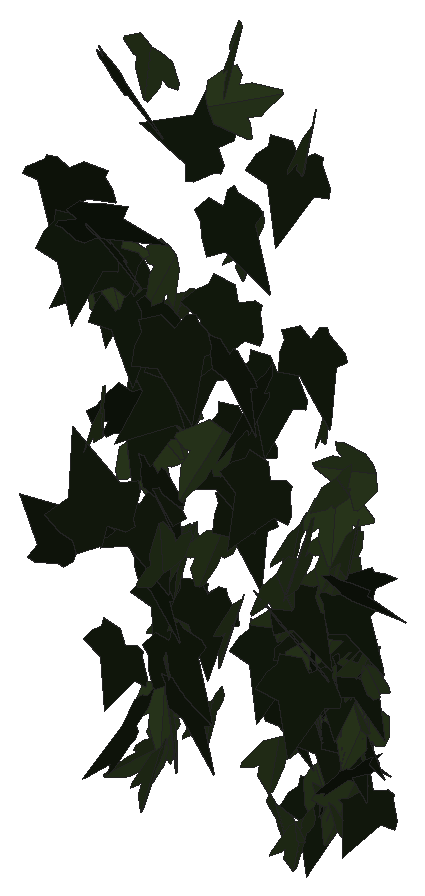
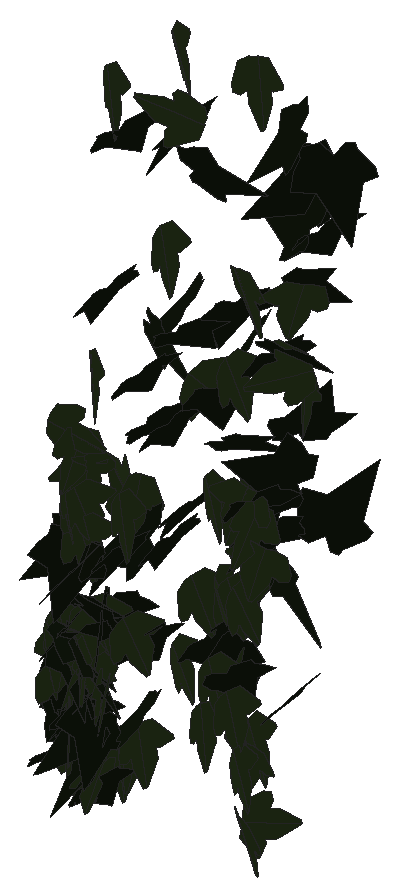
# SketchUp Ruby script. Lengths in inches.
U = 1.inch
M = Sketchup.active_model
def pt(a) = Geom::Point3d.new(a.map { |v| v * U })
def face(e, loops, mat)
  f = e.add_face(loops[0].map { |a| pt(a) })
  loops[1..].each { |l| e.add_face(l.map { |a| pt(a) }).erase! }
  f.material = f.back_material = mat if mat
  f
end
# faces: each face lists its corners as indices into pts; further lists are holes
def faces(e, pts, list, mat = nil) = list.each { |f| face(e, (f[0].is_a?(Array) ? f : [f]).map { |l| l.map { |i| pts[i] } }, mat) }
# xy, xz, yz: faces in a plane at the given z, y or x. An outline is a flat list of corners, or four numbers for a rectangle; further outlines are holes
def ring(l) = l.size == 4 ? [[l[0], l[1]], [l[2], l[1]], [l[2], l[3]], [l[0], l[3]]] : l.each_slice(2).to_a
def flat(e, list, mat, &to3) = list.each { |f| face(e, (f[0].is_a?(Array) ? f : [f]).map { |l| ring(l).map { |u, v| to3.(u, v) } }, mat) }
def xy(e, z, list, mat = nil) = flat(e, list, mat) { |x, y| [x, y, z] }
def xz(e, y, list, mat = nil) = flat(e, list, mat) { |x, z| [x, y, z] }
def yz(e, x, list, mat = nil) = flat(e, list, mat) { |y, z| [x, y, z] }
def lines(e, pts, list) = list.each { |a, b| e.add_line(pt(pts[a]), pt(pts[b])) }
# prism: a flat outline (further loops are holes) pulled along v
def prism(e, loops, v, mat = nil)
  f = face(e, loops, mat); d = Geom::Vector3d.new(v.map { |x| x * U })
  f.pushpull(f.normal.samedirection?(d) ? d.length : -d.length)
end
def box(e, o, s, mat = nil) = prism(e, [[o, [o[0] + s[0], o[1], o[2]], [o[0] + s[0], o[1] + s[1], o[2]], [o[0], o[1] + s[1], o[2]]]], [0, 0, s[2]], mat)
def at(x, y, z, deg = 0) = Geom::Transformation.translation(pt([x, y, z])) * Geom::Transformation.rotation(ORIGIN, Z_AXIS, deg.degrees)
def axes(o, x, y, z) = Geom::Transformation.new([*x, 0, *y, 0, *z, 0, *pt(o).to_a, 1])
def part(name) = M.definitions.add(name)
# library, detail: a bought-in or finely detailed component or shape, given as its bounding box
def library(name, o, s) = part(name).tap { |d| box(d.entities, o, s) }
def detail(e, o, s) = box(e.add_group.entities, o, s)
def put(e, d, t, mat = nil) = e.add_instance(d, t).tap { |i| i.material = mat if mat }
def group(e, t, mat = nil) = e.add_group.tap { |g| g.transformation = t; g.material = mat if mat }.entities
root = M.entities
M.materials.add("efeu1").color = [18, 25, 13]
M.materials.add("efeu2").color = [43, 57, 29]
c1 = part("ivyleaf_9")
p = [[1.54,2.16,1.25],[1.36,2.04,1.19],[-0.21,0.99,0.68],[-0.71,1.11,0.82],[-0.85,0.86,0.67],[-0.8,0.17,0.21],
  [-0.9,-0.01,0.1],[-0.67,-0.16,-0.02],[-0.08,-0.08,-0.05],[-0.03,-0.6,-0.4],[0.65,-0.88,-0.66],[0.83,-0.6,-0.49],
  [1.29,-0.42,-0.43],[1.8125,-0.07,-0.26],[1.21,0.44,0.15]]
faces(c1.entities,p,[[0,1,2,3,4,5,6,7,8,9,10,11,12,13,14]],"efeu1")
c2 = part("ivyleaf_10")
p = [[0,0.5,-0.03],[-0.0625,2.02,-0.43],[-0.19,2.01,-0.46],[-0.54,1.05,-0.29],[-0.52,0.625,-0.18],[-0.83,0.76,-0.28],
  [-1.16,0.64,-0.33],[-1.15,0.33,-0.24],[-0.77,-0.39,0.02],[-0.3,-0.51,0.16],[0.04,-0.48,0.23],[-0.02,2.01,-0.4375],
  [-0.06,2.01,-0.43],[0.04,-0.49,0.23],[0.67,-0.49,0.14],[1.38,0.36,-0.2],[1.375,0.51,-0.24],[0.81,0.65,-0.19],
  [0.62,0.59,-0.15],[0.6,1.09,-0.28],[0.5,1.23,-0.31]]
faces(c2.entities,p,[[0,1,2,3,4,5,6,7,8,9,10],[11,12,0,13,14,15,16,17,18,19,20]],"efeu2")
put(root,c1,axes([520.66,128.22,263.75],[-0.69365,-0.67132,-0.50091],[0.59941,0.05642,-0.90568],[0.58505,-0.85375,0.33402]))
put(root,c2,axes([520.98,130.83,246.47],[0.29708,-0.97872,0.03394],[0.01857,-0.02983,-1.02277],[0.97913,0.29752,0.0091]))
put(root,c2,axes([521.33,129.46,243.19],[-0.16336,0.40857,-0.92125],[-0.63007,-0.76979,-0.22967],[-0.78654,0.5318,0.37532]))
put(root,c2,axes([520.625,129.71,255.22],[0.91836,0.41459,0.34556],[0.25749,0.26283,-0.99965],[-0.47434,0.94536,0.12638]))
put(root,c2,axes([521,130.48,243.49],[0.86834,-0.61453,-0.01149],[-0.00928,0.00678,-1.0638],[0.61457,0.86839,0.00017]))
put(root,c2,axes([520.42,127.77,262.62],[0.32861,0.02903,1.02903],[0.67094,0.81321,-0.2372],[-0.78076,0.71104,0.22926]))
put(root,c1,axes([521.42,124.74,253.9],[0.43717,0.15121,1.08821],[-1.00297,-0.42313,0.46172],[0.44845,-1.09374,-0.02818]))
put(root,c2,axes([521.11,129.59,256.77],[-0.27803,-0.8168,-0.63572],[0.2236,0.59531,-0.86267],[1.01059,-0.35643,0.01598]))
put(root,c1,axes([520.92,128.12,247.9],[-0.16291,-0.90011,0.48411],[0.07985,-0.49993,-0.90266],[1.01891,-0.10474,0.14814]))
put(root,c1,axes([520.78,127.61,257.58],[0.30082,-0.03966,1.04482],[0.88917,0.58171,-0.23392],[-0.5501,0.91857,0.19325]))
put(root,c1,axes([521.27,129.5625,257.41],[-0.45716,-0.971,-0.0412],[0.00221,0.04449,-1.0731],[0.97187,-0.45685,-0.01694]))
put(root,c2,axes([521.58,129.97,253.13],[0.01932,-0.99801,0.34488],[0.00807,-0.34479,-0.9982],[1.05589,0.0209,0.00132]))
put(root,c1,axes([521.83,123.84,269.89],[0.53807,0.6933,-0.78828],[-0.48033,-0.62504,-0.8776],[-0.93345,0.72127,-0.0028]))
put(root,c2,axes([521.625,130.52,248.66],[-0.09822,-1.03062,0.0625],[0.00455,-0.06321,-1.03524],[1.03251,-0.09776,0.01051]))
put(root,c1,axes([521.91,126.54,265.4375],[-0.75241,-0.6843,0.4398],[-0.33722,-0.28278,-1.01692],[0.74025,-0.82436,-0.01624]))
put(root,c2,axes([521.37,126.44,265.23],[0.69116,0.81659,0.26113],[0.16323,0.20395,-1.0698],[-0.84164,0.71014,0.00697]))
put(root,c1,axes([521.13,126.97,272.73],[1.04056,-0.52413,-0.14017],[-0.12231,0.06878,-1.16509],[0.52859,1.04771,0.00636]))
put(root,c2,axes([521.61,129.64,257.48],[0.99003,0.20389,0.3712],[0.28016,0.3925,-0.9628],[-0.31761,0.98179,0.30782]))
put(root,c1,axes([521.94,130.27,249.84],[-0.53362,-0.89248,-0.01376],[0.01586,0.00655,-1.03979],[0.89245,-0.53376,0.01024]))
put(root,c1,axes([521.81,127.56,262.87],[-0.14103,-1.05826,-0.18674],[-0.01066,0.18971,-1.06704],[1.07456,-0.13701,-0.0351]))
put(root,c2,axes([521.95,129,245.91],[1.00038,-0.09883,0.26611],[0.26139,-0.05949,-1.00473],[0.11072,1.03346,-0.03239]))
put(root,c1,axes([521.99,124.53,266.91],[-0.20059,-1.13323,0.06662],[0.01428,-0.07017,-1.15055],[1.1351,-0.19938,0.02625]))
put(root,c2,axes([522.7,129.0625,252.7],[-0.23547,-0.99051,0.24855],[0.02076,-0.25966,-1.01512],[1.02101,-0.22315,0.07796]))
put(root,c2,axes([522.77,124.36,259.98],[0.27143,-0.85202,-0.61381],[-0.12326,0.60376,-0.89256],[1.04284,0.29312,0.05427]))
put(root,c1,axes([522.05,128.76,255.12],[0.49208,-0.89724,0.28373],[0.11153,-0.26232,-1.02295],[0.9344,0.50382,-0.02732]))
put(root,c2,axes([522.74,129.02,262.42],[0.02047,-1.05918,0.27122],[0.01003,-0.27107,-1.05937],[1.09331,0.02232,0.00464]))
put(root,c2,axes([522.9,130,249.48],[-0.01941,-1.03805,0.06821],[-0.01225,-0.06799,-1.03817],[1.04021,-0.02017,-0.01095]))
put(root,c1,axes([523.125,128.75,259.08],[-0.90533,-0.4986,0.31147],[-0.12446,-0.3964,-0.9963],[0.57456,-0.87149,0.27497]))
put(root,c1,axes([522.55,127.07,254.74],[-0.09928,-0.9378,-0.60059],[0.18853,0.58011,-0.93699],[1.09756,-0.18448,0.10663]))
put(root,c2,axes([522.92,128.41,245.82],[-0.53142,0.79284,-0.44341],[0.16062,-0.42361,-0.94994],[-0.8941,-0.54734,0.09289]))
put(root,c1,axes([522.3,124.9,267.1],[0.56545,-0.74923,0.57769],[0.45767,-0.3724,-0.93094],[0.82801,0.71748,0.12006]))
put(root,c1,axes([522.48,127.71,251.79],[0.54406,-0.82297,0.36363],[0.19085,-0.30971,-0.98649],[0.87925,0.57646,-0.01088]))
put(root,c2,axes([523.12,129.2,252.78],[0.50242,-0.88255,0.4192],[0.23127,-0.35056,-1.01522],[0.94928,0.55251,0.02547]))
put(root,c2,axes([523.7,126.32,274.21],[-1.05601,0.10997,0.37654],[-0.38258,-0.04991,-1.05838],[-0.08663,-1.12002,0.08413]))
put(root,c1,axes([522.8,123.29,268.45],[1.0075,0.36353,0.53751],[0.491,0.22194,-1.07042],[-0.42426,1.12014,0.03765]))
put(root,c2,axes([523.75,127.1,265.24],[0.90178,-0.5393,-0.40378],[-0.32362,0.24495,-1.04993],[0.59089,0.9572,0.04119]))
put(root,c2,axes([523.64,126.56,244.98],[0.28969,-1.07798,0.08466],[0.02297,-0.08149,-1.11623],[1.08105,0.2906,0.00103]))
put(root,c2,axes([523.65,129.22,256.95],[0.36565,-1.00278,-0.06325],[-0.01492,0.06188,-1.06734],[1.00466,0.36588,0.00716]))
put(root,c1,axes([523.08,127.37,262.98],[0.67045,-0.87574,-0.1732],[-0.11254,0.13197,-1.10288],[0.88559,0.67977,-0.00902]))
put(root,c1,axes([524.24,122.92,256.6],[-0.89709,-0.79083,0.33482],[0.25533,0.21668,1.19588],[-0.81995,0.93269,0.00608]))
put(root,c2,axes([523.95,129.71,252.68],[-0.24691,-0.98046,0.29137],[-0.06406,-0.28433,-1.01105],[1.02083,-0.25499,0.00702]))
put(root,c2,axes([523.92,127.15,248.42],[-0.61153,0.90955,0.26559],[-0.15359,0.21676,-1.096],[-0.935,-0.63049,0.00634]))
put(root,c1,axes([523.85,128.57,261.02],[-0.35087,-0.99722,-0.25343],[0.06088,0.24717,-1.05688],[1.02712,-0.35531,-0.02393]))
put(root,c1,axes([523.76,129.42,250.39],[0.00275,-1.03963,-0.01107],[0.00009,0.01107,-1.03963],[1.03969,0.00275,0.00012]))
put(root,c1,axes([525.1,128.18,270.13],[-0.62836,0.24693,0.89941],[-0.84084,0.31932,-0.67511],[-0.40361,-1.04967,0.0062]))
put(root,c2,axes([524.39,128.75,246.375],[0.03982,-1.0123,-0.20358],[-0.02534,0.20271,-1.01294],[1.03226,0.04403,-0.01701]))
put(root,c2,axes([524.42,130.21,249.73],[0.36116,-1.00756,0.23911],[0.08739,-0.22267,-1.07031],[1.03185,0.37152,0.00695]))
put(root,c1,axes([523.8125,127.26,249.4375],[-0.22829,-0.26158,-1.0719],[0.97054,0.47307,-0.32215],[0.52484,-0.98858,0.12947]))
put(root,c1,axes([524.17,129.66,256.42],[0.33191,-0.96504,-0.31118],[0.05424,0.34386,-1.00852],[1.01252,0.29793,0.15603]))
put(root,c2,axes([524.61,125.9,253.64],[-0.12168,-1.0582,-0.41002],[-0.05161,-0.40678,1.06516],[-1.13368,0.1321,-0.00448]))
put(root,c1,axes([524.96,126.05,263.32],[-0.07993,-1.07471,-0.41201],[0.1002,0.40493,-1.0757],[1.14661,-0.1103,0.06528]))
put(root,c1,axes([525.38,129.02,263.27],[-0.63674,-0.87552,0.14843],[0.03463,-0.20698,-1.07237],[0.88734,-0.62019,0.14836]))
put(root,c1,axes([524.75,126.78,247.83],[0.5755,-0.91051,0.29425],[0.15124,-0.2525,-1.07712],[0.94485,0.59501,-0.00681]))
put(root,c1,axes([525.2,129.75,254.54],[0.19746,-1.03466,-0.14421],[-0.00544,0.14574,-1.05311],[1.04465,0.19633,0.02178]))
put(root,c1,axes([526.55,121.6875,249.41],[-0.91715,0.88546,-0.13495],[0.08666,-0.10452,-1.27475],[-0.89148,-0.92112,0.01492]))
put(root,c2,axes([526.375,128.66,266.79],[0.12395,-1.09728,-0.09636],[-0.00102,0.09685,-1.10421],[1.1015,0.12356,0.00982]))
put(root,c2,axes([526.39,127.77,275.14],[0.60274,-0.96262,0.13018],[0.10674,-0.08665,-1.13489],[0.9655,0.61052,0.04419]))
put(root,c2,axes([525.61,128.07,272.18],[0.32853,0.0329,-1.08242],[1.06871,0.17281,0.32962],[0.17488,-1.1179,0.0191]))
put(root,c2,axes([526.65,130.51,250.2],[-0.3163,-0.90197,0.36508],[-0.08665,-0.35625,-0.95523],[0.96919,-0.32622,0.03375]))
put(root,c1,axes([526.17,128.63,258.72],[-0.05839,-1.07694,0.07568],[-0.0009,-0.07574,-1.07851],[1.07959,-0.05831,0.0032]))
put(root,c2,axes([526.6875,126.13,259.3],[-0.31224,-0.75686,0.82967],[0.10659,-0.87723,-0.76012],[1.11796,-0.12775,0.30419]))
put(root,c2,axes([526.74,129.73,245.15],[-0.28879,-0.98611,0.05415],[0.01285,-0.06016,-1.02711],[0.98751,-0.28759,0.0292]))
put(root,c1,axes([526.08,130.45,246.57],[0.60078,-0.8126,0.0376],[0.0895,0.01958,-1.00711],[0.80853,0.60163,0.08355]))
put(root,c1,axes([526.68,129.7,249.34],[-0.23979,-1.0029,0.13058],[-0.0172,-0.13014,-1.03108],[1.01122,-0.24003,0.01343]))
put(root,c1,axes([527.11,129.22,260.87],[-0.14846,-1.06241,0.14109],[0.02313,-0.14558,-1.07188],[1.07149,-0.14406,0.04269]))
put(root,c1,axes([527.01,126.69,262.69],[0.49881,-0.93714,0.27791],[0.12604,-0.24773,-1.06161],[0.96932,0.51446,-0.00497]))
put(root,c1,axes([527.92,130.91,246.01],[0.19984,0.98848,0.13533],[-0.0299,0.14388,-1.00685],[-0.99726,0.19376,0.0573]))
put(root,c2,axes([528.01,129.22,254.63],[0.15792,-1.0379,-0.15194],[-0.02443,0.14997,-1.04984],[1.04867,0.15979,-0.00157]))
put(root,c2,axes([528.11,130.15,247.08],[-0.63077,0.74963,0.28405],[-0.24286,0.16575,-0.97675],[-0.76397,-0.67162,0.07598]))
put(root,c1,axes([528.29,126.93,261.47],[-0.88591,0.51029,-0.44101],[0.35257,-0.27026,-1.02096],[-0.57496,-0.95199,0.05345]))
put(root,c2,axes([527.84,130.85,243.76],[0.06975,0.97976,0.17504],[0.02434,0.17374,-0.98217],[-0.99497,0.07293,-0.01175]))
put(root,c2,axes([528.27,130.24,247.34],[-0.48612,0.79816,0.41138],[-0.36738,0.25006,-0.91929],[-0.81934,-0.58568,0.16813]))
put(root,c2,axes([528.25,128.1,243.62],[-0.93544,0.37737,0.11416],[-0.09969,0.05797,-1.00856],[-0.38145,-0.9406,-0.01635]))
put(root,c1,axes([528.12,127.47,257.57],[-0.43556,-0.90485,0.38544],[-0.07696,-0.3889,-0.99993],[0.9805,-0.43247,0.09274]))
put(root,c1,axes([528.88,130.3,250.35],[-0.96933,0.1802,0.34614],[-0.35178,-0.0023,-0.98393],[-0.16892,-1.02927,0.06279]))
put(root,c1,axes([528.11,130.74,242.98],[-0.26148,-0.95649,0.06892],[-0.02066,-0.06581,-0.99158],[0.95874,-0.26228,-0.00257]))
put(root,c1,axes([528.09,131.0625,244.46],[0.89294,-0.17285,-0.43266],[-0.38957,0.23605,-0.89829],[0.25557,0.96375,0.14242]))
put(root,c1,axes([528.66,129.46,250.3125],[0.32773,-0.16783,-0.99526],[-0.89975,0.42556,-0.36805],[0.45733,0.95752,-0.01087]))
put(root,c1,axes([528.91,130.56,248.57],[-0.75022,0.69807,-0.0899],[0.07732,-0.04886,-1.02463],[-0.69958,-0.75401,-0.01684]))
put(root,c1,axes([528.12,125.02,269.9375],[0.499,-0.95515,-0.51361],[-0.12103,0.51279,-1.07121],[1.0777,0.49984,0.11751]))
put(root,c1,axes([528.2,130.85,245.57],[1.01626,0.05111,0.00473],[-0.00527,0.19729,-0.99823],[-0.05106,0.99693,0.1973]))
put(root,c1,axes([528.34,128.8,252.47],[0.33864,-0.88892,-0.4643],[-0.06217,0.47051,-0.94615],[1.00095,0.32996,0.09832]))
put(root,c2,axes([528.91,128.3,243.2],[-0.00351,-1.0242,-0.09739],[-0.00653,0.09741,-1.02419],[1.0288,-0.00288,-0.00683]))
put(root,c2,axes([528.85,130.72,247.84],[0.93857,0.35799,-0.21603],[-0.23714,0.01852,-0.99958],[-0.34437,0.96294,0.09954]))
put(root,c2,axes([529.05,129.75,249.91],[-0.62388,-0.76186,0.3421],[-0.06126,-0.38412,-0.96716],[0.83289,-0.59893,0.18511]))
put(root,c2,axes([528.96,130.82,247.34],[-0.83246,0.57744,0.12979],[-0.11102,0.06767,-1.01309],[-0.58134,-0.83979,0.00761]))
put(root,c1,axes([528.6875,130.89,246.14],[-0.30826,-0.95385,-0.18757],[0.05626,0.17894,-1.00243],[0.97049,-0.31335,-0.00147]))
put(root,c2,axes([528.24,130.49,248.52],[0.63782,0.18426,0.79639],[0.68448,0.43181,-0.6481],[-0.44685,0.92444,0.14399]))
put(root,c2,axes([529.32,129.52,243.62],[-0.83332,0.29268,0.4772],[-0.46175,0.12447,-0.88267],[-0.3165,-0.95218,0.0313]))
put(root,c1,axes([529.12,130.47,250.7],[-0.94428,-0.38036,-0.19061],[0.22823,-0.06128,-1.00838],[0.35905,-0.96137,0.13969]))
put(root,c2,axes([529.03,126.91,254.11],[-0.1584,-0.92289,-0.52642],[0.08794,0.51902,-0.93638],[1.05882,-0.18117,-0.00098]))
put(root,c1,axes([528.82,128.3125,270.71],[-0.34893,-1.06136,0.07986],[0.01499,-0.08894,-1.11646],[1.06426,-0.34673,0.04191]))
put(root,c1,axes([528.27,127.41,252.39],[0.95277,-0.61478,0.27507],[0.2356,-0.1422,-1.13387],[0.63096,0.98144,0.00802]))
put(root,c1,axes([529.63,130.54,249.25],[-0.65613,0.74356,-0.2908],[0.00602,-0.37177,-0.9642],[-0.79838,-0.61388,0.23171]))
put(root,c2,axes([529.0625,130.71,247.5625],[-0.31793,0.92073,-0.32361],[0.00176,-0.33981,-0.96854],[-0.97594,-0.30056,0.10367]))
put(root,c2,axes([529.32,130.72,245.91],[0.39681,-0.8868,-0.49781],[-0.0562,0.51443,-0.9612],[1.01542,0.37502,0.14134]))
put(root,c1,axes([528.77,131.07,246.21],[0.35702,-0.94576,-0.07128],[0.00421,0.07774,-1.01042],[0.94844,0.35567,0.03131]))
put(root,c1,axes([529.63,130.33,248.375],[-0.25779,0.99678,0.00182],[0.009,0.00421,-1.02953],[-0.99675,-0.25777,-0.00977]))
put(root,c2,axes([529.3125,130.57,244.05],[0.22597,-0.96264,-0.24983],[0.00061,0.25633,-0.98714],[0.99453,0.21856,0.05737]))
put(root,c2,axes([529.43,129.95,253.36],[-0.32838,-0.9717,0.2211],[-0.02802,-0.22369,-1.02474],[0.99614,-0.32661,0.04406]))
put(root,c1,axes([529.07,130.56,249.25],[-0.36644,-0.93447,-0.21815],[0.11877,0.18755,-1.0029],[0.95221,-0.38301,0.04115]))
put(root,c2,axes([529.47,129.21,260.44],[0.4661,-0.89201,-0.40491],[-0.08629,0.40928,-1.00096],[0.9758,0.46226,0.10489]))
put(root,c1,axes([529.31,128.29,249.57],[-0.59684,-0.8177,-0.22652],[0.10953,0.20038,-1.01194],[0.8414,-0.60611,-0.02895]))
put(root,c2,axes([529.33,127.45,253.91],[0.50192,-1.01047,0.33531],[-0.15162,0.29908,1.12826],[-1.0538,-0.52431,-0.00262]))
put(root,c2,axes([529.65,129.83,254.67],[-0.30394,-0.94095,0.36589],[-0.03732,-0.37137,-0.98606],[1.00889,-0.29721,0.07375]))
put(root,c2,axes([529.62,130.79,248.85],[-1.02437,-0.06006,0.02293],[-0.02235,-0.01058,-1.02609],[0.06028,-1.02457,0.00925]))
put(root,c2,axes([529.4375,130.55,247.33],[-0.85338,0.51004,-0.19264],[0.14278,-0.13624,-0.99325],[-0.52618,-0.86417,0.0429]))
put(root,c1,axes([529.57,130.14,252.72],[0.50099,0.91234,-0.0691],[-0.03438,-0.05995,-1.04084],[-0.9143,0.50216,0.00127]))
put(root,c2,axes([529.69,127.83,272.4],[0.31611,-1.03952,-0.31751],[-0.0827,0.3067,-1.08648],[1.08378,0.32661,0.00971]))
put(root,c1,axes([528.86,130.85,246.86],[-0.06714,-0.01462,-1.01938],[0.96732,0.32171,-0.06832],[0.32195,-0.96962,-0.0073]))
put(root,c2,axes([529.75,130.08,244.13],[-0.23862,-0.88078,0.47831],[-0.0044,-0.49076,-0.90589],[1.00227,-0.21185,0.10991]))
put(root,c2,axes([530.47,129.94,257.73],[0.25248,-0.01406,-1.02872],[-1.01067,0.19468,-0.25071],[0.19238,1.0412,0.03298]))
put(root,c2,axes([529.67,130.64,248.8],[-0.92901,0.37643,-0.22818],[0.14958,-0.23123,-0.99045],[-0.41399,-0.92826,0.15419]))
put(root,c2,axes([529.61,129.5,256.15],[0.62022,0.83815,-0.10849],[-0.05986,-0.09067,-1.04266],[-0.84302,0.62308,-0.00578]))
put(root,c1,axes([530.15,129.78,245.29],[-0.24765,0.88747,-0.4298],[-0.00395,-0.44404,-0.91459],[-0.98606,-0.22111,0.11161]))
put(root,c2,axes([529.89,130.56,249.43],[-0.22532,-0.99096,0.18723],[0.00008,-0.19187,-1.01538],[1.00849,-0.22139,0.04191]))
put(root,c2,axes([529.76,129.64,257.16],[-0.35486,-0.86746,-0.47866],[0.21382,0.4294,-0.93671],[0.96741,-0.41311,0.03145]))
put(root,c1,axes([529.47,128.31,263.45],[0.18811,-1.06563,-0.18462],[0.00407,0.18809,-1.0815],[1.08149,0.18464,0.03618]))
put(root,c2,axes([530.03,130.72,249.46],[0.05358,-0.98,0.30182],[0.02069,-0.30113,-0.98146],[1.02522,0.05729,0.00404]))
put(root,c1,axes([529.45,130.26,251.94],[0.4974,-0.88998,-0.24287],[0.01283,0.28257,-1.00918],[0.92243,0.47597,0.145]))
put(root,c2,axes([530.0625,129.92,254.99],[0.23142,-1.01871,-0.1879],[-0.02126,0.18782,-1.04446],[1.03568,0.23148,0.02055]))
put(root,c2,axes([530.15,130.58,247.1],[-0.60466,-0.67893,0.45613],[-0.02261,-0.55315,-0.85331],[0.81762,-0.5174,0.31373]))
put(root,c1,axes([529.41,129.65,252.84],[1.01806,0.04602,0.24134],[0.23203,0.15818,-1.00893],[-0.08079,1.03425,0.14357]))
put(root,c1,axes([529.69,130.6,249.26],[0.45767,-0.8749,-0.28653],[-0.14604,0.24693,-0.98727],[0.90897,0.48019,-0.01436]))
put(root,c1,axes([530.14,130.95,243.9],[-0.38612,-0.87672,0.31365],[0.05814,-0.36158,-0.93914],[0.92932,-0.34165,0.18907]))
